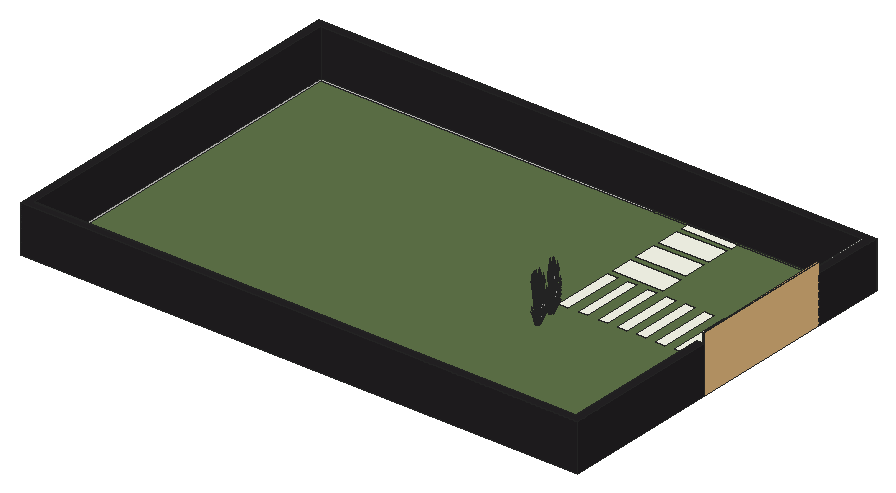
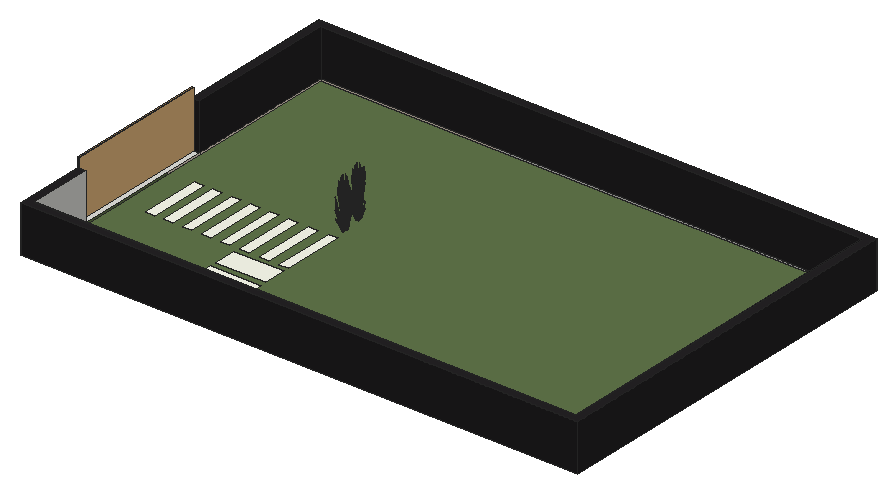
# SketchUp Ruby script. Lengths in inches.
U = 1.inch
M = Sketchup.active_model
def pt(a) = Geom::Point3d.new(a.map { |v| v * U })
def face(e, loops, mat)
  f = e.add_face(loops[0].map { |a| pt(a) })
  loops[1..].each { |l| e.add_face(l.map { |a| pt(a) }).erase! }
  f.material = f.back_material = mat if mat
  f
end
# faces: each face lists its corners as indices into pts; further lists are holes
def faces(e, pts, list, mat = nil) = list.each { |f| face(e, (f[0].is_a?(Array) ? f : [f]).map { |l| l.map { |i| pts[i] } }, mat) }
# xy, xz, yz: faces in a plane at the given z, y or x. An outline is a flat list of corners, or four numbers for a rectangle; further outlines are holes
def ring(l) = l.size == 4 ? [[l[0], l[1]], [l[2], l[1]], [l[2], l[3]], [l[0], l[3]]] : l.each_slice(2).to_a
def flat(e, list, mat, &to3) = list.each { |f| face(e, (f[0].is_a?(Array) ? f : [f]).map { |l| ring(l).map { |u, v| to3.(u, v) } }, mat) }
def xy(e, z, list, mat = nil) = flat(e, list, mat) { |x, y| [x, y, z] }
def xz(e, y, list, mat = nil) = flat(e, list, mat) { |x, z| [x, y, z] }
def yz(e, x, list, mat = nil) = flat(e, list, mat) { |y, z| [x, y, z] }
def lines(e, pts, list) = list.each { |a, b| e.add_line(pt(pts[a]), pt(pts[b])) }
# prism: a flat outline (further loops are holes) pulled along v
def prism(e, loops, v, mat = nil)
  f = face(e, loops, mat); d = Geom::Vector3d.new(v.map { |x| x * U })
  f.pushpull(f.normal.samedirection?(d) ? d.length : -d.length)
end
def box(e, o, s, mat = nil) = prism(e, [[o, [o[0] + s[0], o[1], o[2]], [o[0] + s[0], o[1] + s[1], o[2]], [o[0], o[1] + s[1], o[2]]]], [0, 0, s[2]], mat)
def at(x, y, z, deg = 0) = Geom::Transformation.translation(pt([x, y, z])) * Geom::Transformation.rotation(ORIGIN, Z_AXIS, deg.degrees)
def axes(o, x, y, z) = Geom::Transformation.new([*x, 0, *y, 0, *z, 0, *pt(o).to_a, 1])
def part(name) = M.definitions.add(name)
# library, detail: a bought-in or finely detailed component or shape, given as its bounding box
def library(name, o, s) = part(name).tap { |d| box(d.entities, o, s) }
def detail(e, o, s) = box(e.add_group.entities, o, s)
def put(e, d, t, mat = nil) = e.add_instance(d, t).tap { |i| i.material = mat if mat }
def group(e, t, mat = nil) = e.add_group.tap { |g| g.transformation = t; g.material = mat if mat }.entities
root = M.entities
M.materials.add("Concrete_04_1K").color = [254, 255, 241]
M.materials.add("LightPink_Translucent").color = [144, 107, 117]
M.materials["LightPink_Translucent"].alpha = 0.75
M.materials.add("Marble_07_1K").color = [36, 34, 36]
M.materials.add("Roofing_01_1K1").color = [234, 220, 203]
M.materials.add("Roofing_02_1K").color = [97, 118, 74]
c1 = part("blade")
p = [[2.15,0.21,22],[0,0.17,0],[0.09,0.45,0],[2.18,0.31,22],[2.29,0.31,22],[0.38,0.45,0],
  [2.48,0.24,33],[2.49,0.24,33],[2.48,0.22,33]]
faces(c1.entities,p,[[0,1,2,3],[4,5,2,3],[6,3,4,7],[8,0,3,6]])
c2 = part("seeds")
p = [[0.3,-0.1,1.38],[-0.01,-0.03,1.59],[-0.01,-0.03,0.03],[0.14,-0.07,-0.07],[0.29,-0.03,3],[0.15,0.01,3.11]]
faces(c2.entities,p,[[0,1,2,3],[1,0,4,5]],"LightPink_Translucent")
c3 = part("blade with seeds")
put(c3.entities,c1,at(0,0,0))
put(c3.entities,c2,axes([2.4,0.25,30.99],[1.5799,-0.05474,1.17369],[-0.12525,1.92788,0.29478],[-0.07173,-0.02425,1.56792]))
c4 = library("Modern+Gate+1",[0,0,0],[118.11,1.97,78.74])
xy(root,-4,[[9,9,621,413.18]],"Roofing_02_1K")
xy(root,-2,[[0,0,0,422.18,630,422.18,630,341.02,621,341.02,621,413.18,9,413.18,9,9,621,9,621,179.2,630,179.2,630,0],[621,179.2,630,341.02]])
xy(root,0,[[428.41,225.85,438.8125,295.18],[450.39,225.85,460.8,295.18],[473.09,225.85,483.5,295.18],[494.45,225.85,504.85,295.18],[515.86,225.85,526.26,295.18],
  [537.75,225.85,548.15,295.18],[559.25,225.85,569.66,295.18],[579.86,225.85,590.27,295.18],[428.21,302.1,484.72,327.6],[428.21,335.07,484.72,360.33],
  [428.21,367.55,484.72,392.98],[428.21,399.17,484.72,408.11]],"Concrete_04_1K")
xy(root,51,[[0,0,630,0,630,179.2,621,179.2,621,9,9,9,9,413.18,621,413.18,621,341.02,630,341.02,630,422.18,0,422.18]],"Marble_07_1K")
xz(root,0,[[0,-2,630,51]],"Marble_07_1K")
xz(root,9,[[9,-4,423,-2]])
xz(root,9,[[9,-2,621,51]],"Marble_07_1K")
xz(root,9,[[423,-4,621,-2]],"Roofing_01_1K1")
xz(root,179.2,[[621,-2,630,51]],"Marble_07_1K")
xz(root,341.02,[[621,-2,630,51]],"Marble_07_1K")
xz(root,413.18,[[9,-4,387,-2]])
xz(root,413.18,[[9,-2,621,51]],"Marble_07_1K")
xz(root,413.18,[[387,-4,621,-2]],"Roofing_02_1K")
xz(root,422.18,[[0,-2,630,51]],"Marble_07_1K")
yz(root,0,[[0,-2,422.18,51]],"Marble_07_1K")
yz(root,9,[[9,-4,413.18,-2]])
yz(root,9,[[9,-2,413.18,51]],"Marble_07_1K")
yz(root,621,[[341.02,-2,413.18,51]])
yz(root,621,[[9,-2,179.2,51]],"Marble_07_1K")
yz(root,621,[[9,-4,179.2,-2],[179.2,-4,225.85,-2]],"Roofing_01_1K1")
yz(root,621,[[225.85,-4,294.89,-2],[294.89,-4,341.02,-2],[341.02,-4,413.18,-2]],"Roofing_02_1K")
yz(root,630,[[0,-2,179.2,51],[341.02,-2,422.18,51]],"Marble_07_1K")
put(root,c3,axes([435.76,185.8,0.29],[-0.04385,-0.62963,-0.25022],[0.45669,-0.03807,-0.43002],[0.08042,-0.08387,1.37348]))
put(root,c3,axes([434.63,185.83,-0.26],[0.26266,-0.34428,-0.26641],[0.26266,0.34428,0.26641],[0,-0.11089,1.19518]))
put(root,c3,axes([434.52,184.18,-0.17],[-0.10855,0.45057,-0.03348],[-0.33409,-0.1386,-0.15179],[-0.05073,-0.0737,0.50065]))
put(root,c3,axes([435.55,186.45,0.29],[-0.42377,-0.26329,-0.25022],[0.20405,-0.55571,-0.43002],[-0.01332,-0.13644,1.37348]))
put(root,c3,axes([434.34,186.23,0.04],[-0.47052,0,0],[0,-0.61671,-0.44382],[0,-0.14046,1.40792]))
put(root,c3,axes([435.7,184.4,-0.26],[0.35106,0.13653,-0.26641],[-0.08839,0.48081,0.26641],[0.07077,-0.05545,1.19518]))
put(root,c3,axes([434.71,186.07,0],[-0.35001,0.46392,0.2645],[-0.35022,-0.45904,-0.31383],[-0.01222,-0.13174,1.41801]))
put(root,c3,axes([435.82,186.29,0.09],[0.42398,0.26744,0.20696],[-0.20405,0.55571,0.43002],[0,-0.1281,1.38067]))
put(root,c3,axes([435.66,187.04,0.1],[0.09973,-0.65385,-0.20149],[0.47288,0.11397,0.44093],[-0.08263,-0.0903,1.34539]))
put(root,c3,axes([433.99,185.59,0.38],[0.24023,-0.03948,0.9878],[-0.15239,0.3479,0.72577],[-0.11872,-0.05219,0.21757]))
put(root,c3,axes([435.68,185.92,0.34],[-0.40861,0.03406,0.38476],[-0.03695,-0.56543,-0.18517],[0.07315,-0.05731,1.23533]))
put(root,c3,axes([434.63,186.33,0.13],[0,0.5518,0.427],[-0.42099,0,0],[0,-0.12568,1.35453]))
put(root,c3,axes([437.58,186.45,2.03],[0.10194,-0.50193,-0.43945],[0.34951,0.17204,-0.34039],[0.14072,-0.04602,0.84085]))
put(root,c3,axes([437.03,184.41,0.04],[0.23526,-0.55293,0],[0.3936,0.30836,-0.44382],[0.08964,0.07023,1.40792]))
put(root,c3,axes([435.62,186.77,-0.1],[-0.22605,-0.46315,-0.38476],[0.34239,-0.32614,0.18517],[-0.07315,-0.05731,1.23533]))
put(root,c3,axes([435.67,186.12,0.03],[0.1636,0.61702,0.39349],[-0.46745,0.21456,0.15441],[0.00571,-0.11338,1.36617]))
put(root,c3,axes([437.96,186.59,-0.3],[-0.24235,0.06622,1.21762],[-0.03858,-0.5271,0.0697],[0.16974,-0.07978,0.69287]))
put(root,c3,axes([438.4,186.125,-0.06],[-0.23329,-0.35284,-0.05579],[0.2555,-0.3233,-0.25298],[0.0724,-0.02276,0.83441]))
put(root,c3,axes([435.59,186.61,0.34],[-0.18257,0.49721,0.38476],[-0.37935,-0.23929,-0.18517],[0,-0.11462,1.23533]))
put(root,c3,axes([436.26,186.17,-0.1],[0,-0.63847,0],[0.47052,0,0],[0,0,1.54332]))
put(root,c3,axes([436.83,184.7,0.13],[-0.35217,-0.2759,0.427],[0.2105,-0.49473,0],[0.08021,0.06284,1.35453]))
put(root,c3,axes([437.52,186.63,2.28],[0.33065,-0.2437,-0.61099],[0.18427,0.50165,0.07373],[0.15976,-0.05699,0.8643]))
put(root,c3,axes([435.42,186.95,-0.23],[-0.39143,-0.09047,-0.53624],[0.0826,-0.55804,-0.14074],[-0.11681,-0.06762,1.18365]))
put(root,c3,axes([436.04,185.77,0.03],[-0.312,0.50076,0.39349],[-0.37066,-0.44204,0.15441],[0.07522,-0.04998,1.36617]))
put(root,c3,axes([436.375,186.67,-0.02],[-0.35001,-0.47494,-0.05273],[0.35022,-0.47523,0],[-0.01222,-0.01659,1.50991]))
put(root,c3,axes([435.49,184.95,0.13],[-0.1087,0.54839,0.15172],[-0.39778,-0.15519,0.30174],[0.06871,-0.00267,1.3795]))
put(root,c3,axes([435.33,185.39,-0.63],[-0.37038,0.22092,1.10879],[-0.11789,-0.63387,0.43083],[0.22743,0.01055,1.26112]))
put(root,c3,axes([436.32,185.55,0.25],[0.07259,-0.49245,0.12452],[0.35466,0.08548,-0.35559],[0.06454,0.05057,1.09]))
put(root,c3,axes([435.71,186.72,0.03],[0.4756,0.11626,0.39349],[-0.09679,0.6566,0.15441],[-0.0695,-0.0634,1.36617]))
put(root,c3,axes([438.22,186.25,-0.72],[-0.01967,-0.08377,1.51654],[0.1364,-0.49004,-0.23168],[0.13759,-0.00705,0.25832]))
put(root,c3,axes([436.17,185.68,0.34],[-0.22605,-0.46315,0.38476],[0.34239,-0.32614,-0.18517],[0.07315,0.05731,1.23533]))
put(root,c3,axes([435,187.8,-0.26],[-0.08839,-0.48081,-0.26641],[0.35106,-0.13653,0.26641],[-0.07077,-0.05545,1.19518]))
put(root,c3,axes([435.46,187.77,0.13],[0.40434,-0.14646,0.15172],[0.09984,0.54504,0.30174],[-0.03606,-0.07941,1.3795]))
put(root,c3,axes([436.29,185.71,0.29],[0.37992,-0.36634,-0.25022],[0.25264,0.51764,-0.43002],[0.09374,0.05257,1.37348]))
put(root,c3,axes([437.8,186.68,1.89],[0.31272,0.15393,-0.30456],[-0.09121,0.44909,0.39319],[0.1259,-0.04118,0.75234]))
put(root,c3,axes([434.91,188.01,-0.26],[-0.35217,-0.2759,-0.427],[0.2105,-0.49473,0],[-0.08021,-0.06284,1.35453]))
put(root,c3,axes([437.25,184.74,-0.26],[0.35217,0.2759,-0.427],[-0.2105,0.49473,0],[0.08021,0.06284,1.35453]))
put(root,c3,axes([436.58,186.31,-0.1],[0.42099,0,0],[0,0.57126,0],[0,0,1.5343]))
put(root,c3,axes([435.86,187.03,0.29],[-0.37992,0.36634,-0.25022],[-0.25264,-0.51764,-0.43002],[-0.09374,-0.05257,1.37348]))
put(root,c3,axes([436.7,184.98,0.13],[-0.40434,0.14646,0.15172],[-0.09984,-0.54504,0.30174],[0.03606,0.07941,1.3795]))
put(root,c3,axes([437.15,184.95,-0.26],[0.08839,0.48081,-0.26641],[-0.35106,0.13653,0.26641],[0.07077,0.05545,1.19518]))
put(root,c3,axes([436.44,186.02,0.05],[-0.4756,-0.11626,0.42311],[0.09679,-0.6566,0.16603],[0.0695,0.0634,1.46899]))
put(root,c3,axes([436.0625,187.64,-0.1],[-0.12277,-0.47573,0],[0.35059,-0.1666,0],[0,0,1.32759]))
put(root,c3,axes([435.83,187.19,0.25],[-0.07259,0.49245,0.12452],[-0.35466,-0.08548,-0.35559],[-0.06454,-0.05057,1.09]))
put(root,c3,axes([436.52,187.58,-0.12],[0.39505,-0.18722,-0.1651],[0.13882,0.53931,0.00007],[0.04361,-0.02069,1.49552]))
put(root,c3,axes([436.66,187.8,0.13],[0.1087,-0.54839,0.15172],[0.39778,0.15519,0.30174],[-0.06871,0.00267,1.3795]))
put(root,c3,axes([436.57,186.56,-0.1],[0.26266,0.35642,0],[-0.26266,0.35642,0],[0,0,1.45569]))
put(root,c3,axes([437.28,186.4,0.13],[-0.29564,-0.40194,0.15172],[0.29793,-0.38985,0.30174],[-0.03265,0.08208,1.3795]))
put(root,c3,axes([436.73,185.8,-0.23],[0.39143,0.09047,-0.53624],[-0.0826,0.55804,-0.14074],[0.11681,0.06762,1.18365]))
put(root,c3,axes([438.46,186.77,0.38],[-0.23249,0.0911,0.9878],[0.10944,-0.37648,0.72577],[0.12334,0.02576,0.21757]))
put(root,c3,axes([435.98,187.86,-0.11],[-0.37935,-0.24773,0],[0.18257,-0.51475,0],[0,0,1.39928]))
put(root,c3,axes([436.29,187.2,0.12],[-0.36743,-0.44413,-0.21665],[0.30918,-0.49872,0.47412],[-0.09894,0.05195,1.44665]))
put(root,c3,axes([435.32,188.05,0.13],[0.35217,0.2759,0.427],[-0.2105,0.49473,0],[-0.08021,-0.06284,1.35453]))
put(root,c3,axes([436.5625,186.14,0.34],[0.18257,-0.49721,0.38476],[0.37935,0.23929,-0.18517],[0,0.11462,1.23533]))
put(root,c3,axes([436.49,186.43,-0.03],[0,0.63816,-0.04848],[-0.47052,0,0],[0,0.02005,1.54256]))
put(root,c3,axes([436.53,185.97,-0.1],[0.22605,0.46315,-0.38476],[-0.34239,0.32614,0.18517],[0.07315,0.05731,1.23533]))
put(root,c3,axes([435.12,188.34,0.04],[-0.23526,0.55293,0],[-0.3936,-0.30836,-0.44382],[-0.08964,-0.07023,1.40792]))
put(root,c3,axes([437.52,186.42,0.13],[0,-0.5518,0.427],[0.42099,0,0],[0,0.12568,1.35453]))
put(root,c3,axes([436.47,186.83,0.34],[0.40861,-0.03406,0.38476],[0.03695,0.56543,-0.18517],[-0.07315,0.05731,1.23533]))
put(root,c3,axes([436.72,186.26,0.25],[0.35059,-0.16092,0.12452],[0.12277,0.45952,-0.35559],[0,0.10113,1.09]))
put(root,c3,axes([436.1,187.11,-0.1],[-0.40861,0.03406,-0.38476],[-0.03695,-0.56543,0.18517],[-0.07315,0.05731,1.23533]))
put(root,c3,axes([438.03,187.375,0.23],[-0.09062,-0.13571,1.22981],[0.11791,-0.44895,-0.26449],[0.18335,0.06082,0.52581]))
put(root,c3,axes([436.41,187.87,-0.1],[0.37935,0.24773,0],[-0.18257,0.51475,0],[0,0,1.5046]))
put(root,c3,axes([436.56,188.42,-0.11],[-0.23233,-0.55486,-0.04422],[0.3936,-0.30836,0.44382],[-0.09699,0.05283,1.40722]))
put(root,c3,axes([436.47,187.08,0.25],[0.278,0.33153,0.12452],[-0.23189,0.37404,-0.35559],[-0.06454,0.05057,1.09]))
put(root,c3,axes([437.19,187.65,2.28],[0.37615,0.01329,-0.61099],[-0.02526,0.55946,0.07373],[0.15935,0.05904,0.8643]))
put(root,c3,axes([436.77,188.1,0.13],[0.35217,-0.2759,0.427],[0.2105,0.49473,0],[-0.08021,0.06284,1.35453]))
put(root,c3,axes([436.27,187.66,-0.03],[0.1636,0.63392,-0.05171],[-0.46745,0.22213,0],[0.00571,0.02214,1.48069]))
put(root,c3,axes([436.45,188.35,-0.26],[-0.35106,-0.13653,-0.26641],[0.08839,-0.48081,0.26641],[-0.07077,0.05545,1.19518]))
put(root,c3,axes([437.81,186.51,0.04],[0.47052,0,0],[0,0.61671,-0.44382],[0,0.14046,1.40792]))
put(root,c3,axes([437.62,186.83,-0.11],[-0.47029,-0.00441,-0.0428],[0,-0.61671,0.42951],[-0.01478,0.14039,1.36183]))
put(root,c3,axes([436.6,186.29,0.29],[0.42377,0.26329,-0.25022],[-0.20405,0.55571,-0.43002],[0.01332,0.13644,1.37348]))
put(root,c3,axes([433.65,188.34,0.38],[0.15682,-0.25009,0.9878],[0.06188,0.39591,0.72577],[-0.11333,0.07089,0.21757]))
put(root,c3,axes([437.42,187.88,1.89],[0.2141,0.34548,-0.30456],[-0.24447,0.32704,0.39319],[0.12421,0.04976,0.75234]))
put(root,c3,axes([437.52,186.92,-0.26],[-0.26266,0.34428,-0.26641],[-0.26266,-0.34428,0.26641],[0,0.11089,1.19518]))
put(root,c3,axes([436.39,186.95,0.29],[0.04385,0.62963,-0.25022],[-0.45669,0.03807,-0.43002],[-0.08042,0.08387,1.37348]))
put(root,c3,axes([436.56,186.71,-0.1],[-0.18257,0.49721,-0.38476],[-0.37935,-0.23929,0.18517],[0,0.11462,1.23533]))
put(root,c3,axes([434.24,187.26,1.89],[-0.32754,0.07886,-0.30456],[-0.08649,-0.45081,0.39319],[-0.09386,0.12109,0.75234]))
put(root,c3,axes([436.12,187.43,-0.23],[-0.25345,0.41475,-0.53624],[-0.31485,-0.37608,-0.14074],[-0.10156,0.10346,1.18365]))
put(root,c3,axes([436.57,188.13,0],[0.47108,0.17935,0.2645],[-0.11785,0.64108,-0.31383],[-0.07797,0.08023,1.41801]))
put(root,c3,axes([436.53,188.57,-0.26],[-0.35217,0.2759,-0.427],[-0.2105,-0.49473,0],[-0.08021,0.06284,1.35453]))
put(root,c3,axes([437.7,186.93,-0.26],[0,0.5518,-0.427],[-0.42099,0,0],[0,0.12568,1.35453]))
put(root,c3,axes([437.17,188.08,0.38],[-0.21187,-0.15866,0.9878],[0.27357,-0.16121,0.72577],[0.07379,0.13656,0.21757]))
put(root,c3,axes([434.51,187.3125,2.03],[0.09666,0.50384,-0.43945],[-0.36608,0.08814,-0.34039],[-0.10491,0.13533,0.84085]))
put(root,c3,axes([436.85,188.48,0.04],[0.23526,0.55293,0],[-0.3936,0.30836,-0.44382],[-0.08964,0.07023,1.40792]))
put(root,c3,axes([437.23,188.67,-0.72],[0.02741,-0.07966,1.51654],[0.34514,-0.23462,-0.23168],[0.10464,0.12143,0.25832]))
put(root,c3,axes([436.65,186.29,0.44],[-0.01028,-0.51954,1.21494],[0.46521,0.13467,0.51441],[-0.11003,0.28429,1.14681]))
put(root,c3,axes([436.77,186.86,-0.2],[0.13798,0.50522,-0.59522],[-0.39745,0.18195,-0.15622],[0.01525,0.17108,1.31385]))
put(root,c3,axes([434.06,188.6,-0.72],[0.05047,0.05513,1.51654],[0.08558,0.51079,-0.23168],[-0.11187,0.10892,0.25832]))
put(root,c3,axes([436.69,188.3,2.03],[0.37131,-0.13117,-0.43945],[0.06495,0.49674,-0.34039],[0.09973,0.14235,0.84085]))
put(root,c3,axes([437.2,188.8,0.29],[-0.2413,-0.01731,0.90352],[0.15935,-0.36755,0.49885],[0.09532,0.13058,0.70873]))
put(root,c3,axes([436.41,187.91,0.23],[0.00664,-0.18292,1.22981],[0.31732,-0.20432,-0.26449],[0.09796,0.21893,0.52581]))
put(root,c3,axes([434.8125,188.3,1.89],[-0.2546,0.29052,-0.30456],[-0.24101,-0.33173,0.39319],[-0.03667,0.16855,0.75234]))
put(root,c3,axes([434.98,189.43,0.38],[-0.00974,-0.3281,0.9878],[0.24334,0.23402,0.72577],[-0.04786,0.15639,0.21757]))
put(root,c3,axes([435.62,188.65,-0.72],[0.0609,-0.03003,1.51654],[0.36632,0.16527,-0.23168],[0.01071,0.18627,0.25832]))
put(root,c3,axes([435.07,188.17,2.3],[0.26937,0.37076,-0.48779],[-0.28456,0.3247,-0.37783],[-0.04099,0.18838,0.93334]))
put(root,c3,axes([434.77,188.72,0.43],[0.34184,-0.09771,0.05596],[0.07859,0.39367,-0.74222],[-0.02167,0.19928,0.6653]))
put(root,c3,axes([435.87,188.53,2.03],[0.3699,0.13833,-0.43945],[-0.12679,0.47426,-0.34039],[0.03392,0.19095,0.84085]))
put(root,c3,axes([435.7,188.82,1.89],[-0.11344,0.42434,-0.30456],[-0.33096,-0.12377,0.39319],[0.03035,0.17085,0.75234]))
put(root,c3,axes([434.98,188,2.59],[-0.00979,0.51041,-0.6782],[-0.4123,-0.03428,0.08184],[-0.04351,0.21623,0.95938]))
put(root,c3,axes([435.73,188.4375,2.28],[0.17959,0.44867,-0.61099],[-0.36969,0.25004,0.07373],[0.042,0.21679,0.8643]))
put(root,c3,axes([434.69,189.14,0.23],[0.11874,-0.08705,1.22981],[0.29317,0.26247,-0.26449],[-0.08726,0.22711,0.52581]))
put(root,c3,axes([434.84,188.72,0.89],[0.00827,-0.28486,1.32737],[0.37184,0.15046,0.18343],[-0.03222,0.30359,0.62678]))
put(root,c3,axes([433.22,207.92,0.23],[-0.10696,0.11169,1.22981],[-0.32033,-0.19549,-0.26449],[0.05938,-0.24312,0.52581]))
put(root,c3,axes([432.74,208.31,2.28],[-0.17959,-0.44867,-0.61099],[0.36969,-0.25004,0.07373],[-0.042,-0.21679,0.8643]))
put(root,c3,axes([432.43,207.3125,-0.72],[-0.06312,0.01988,1.51654],[-0.34903,-0.22379,-0.23168],[0.00586,-0.18666,0.25832]))
put(root,c3,axes([433.48,208.75,2.28],[0.00979,-0.51041,-0.61099],[0.4123,0.03428,0.07373],[0.04351,-0.21623,0.8643]))
put(root,c3,axes([432.83,207.03,0.38],[0.04827,0.32177,0.9878],[-0.26778,-0.17821,0.72577],[0.02882,-0.16476,0.21757]))
put(root,c3,axes([433.4,208.58,2.03],[-0.26937,-0.37076,-0.43945],[0.28456,-0.3247,-0.34039],[0.04099,-0.18838,0.84085]))
put(root,c3,axes([433.97,208.26,-0.72],[-0.05632,-0.04347,1.51654],[-0.14467,-0.48565,-0.23168],[0.09759,-0.13179,0.25832]))
put(root,c3,axes([433.97,209.63,2.28],[0.19655,-0.43539,-0.61099],[0.34443,0.30942,0.07373],[0.11736,-0.15774,0.8643]))
put(root,c3,axes([431.84,208.37,0.04],[-0.23526,-0.55293,0],[0.3936,-0.30836,-0.44382],[0.08964,-0.07023,1.40792]))
put(root,c3,axes([433.96,209.43,2.03],[-0.09666,-0.50384,-0.43945],[0.36608,-0.08814,-0.34039],[0.10491,-0.13533,0.84085]))
put(root,c3,axes([432.16,208.28,-0.26],[0.35217,-0.2759,-0.427],[0.2105,0.49473,0],[0.08021,-0.06284,1.35453]))
put(root,c3,axes([434.25,209.23,0.23],[-0.13443,-0.01634,1.22981],[-0.13772,-0.43844,-0.26449],[0.16514,-0.12403,0.52581]))
put(root,c3,axes([432.58,209.41,-0.23],[0.25345,-0.41475,-0.53624],[0.31485,0.37608,-0.14074],[0.10156,-0.10346,1.18365]))
put(root,c3,axes([434.41,208.43,0.38],[-0.12533,0.28089,0.9878],[-0.10773,-0.37739,0.72577],[0.10352,-0.09457,0.21757]))
put(root,c3,axes([432.14,210.14,-0.1],[0.18257,-0.49721,-0.38476],[0.37935,0.23929,0.18517],[0,-0.11462,1.23533]))
put(root,c3,axes([432.31,209.89,0.29],[-0.04385,-0.62963,-0.25022],[0.45669,-0.03807,-0.43002],[0.08042,-0.08387,1.37348]))
put(root,c3,axes([432.25,208.5,-0.26],[0.35106,0.13653,-0.26641],[-0.08839,0.48081,0.26641],[0.07077,-0.05545,1.19518]))
put(root,c3,axes([432.37,210.39,0.09],[0.42398,0.26744,0.20696],[-0.20405,0.55571,0.43002],[0,-0.1281,1.38067]))
put(root,c3,axes([432.23,210.01,0.34],[-0.40861,0.03406,0.38476],[-0.03695,-0.56543,-0.18517],[0.07315,-0.05731,1.23533]))
put(root,c3,axes([434.13,210.55,2.03],[0.10194,-0.50193,-0.43945],[0.34951,0.17204,-0.34039],[0.14072,-0.04602,0.84085]))
put(root,c3,axes([433.58,208.51,0.04],[0.23526,-0.55293,0],[0.3936,0.30836,-0.44382],[0.08964,0.07023,1.40792]))
put(root,c3,axes([432.22,210.22,0.03],[0.1636,0.61702,0.39349],[-0.46745,0.21456,0.15441],[0.00571,-0.11338,1.36617]))
put(root,c3,axes([434.5,210.69,-0.3],[-0.24235,0.06622,1.21762],[-0.03858,-0.5271,0.0697],[0.16974,-0.07978,0.69287]))
put(root,c3,axes([434.94,210.22,-0.06],[-0.23329,-0.35284,-0.05579],[0.2555,-0.3233,-0.25298],[0.0724,-0.02276,0.83441]))
put(root,c3,axes([432.8,210.27,-0.1],[0,-0.63847,0],[0.47052,0,0],[0,0,1.54332]))
put(root,c3,axes([433.375,208.79,0.13],[-0.35217,-0.2759,0.427],[0.2105,-0.49473,0],[0.08021,0.06284,1.35453]))
put(root,c3,axes([434.0625,210.73,2.28],[0.33065,-0.2437,-0.61099],[0.18427,0.50165,0.07373],[0.15976,-0.05699,0.8643]))
put(root,c3,axes([432.58,209.87,0.03],[-0.312,0.50076,0.39349],[-0.37066,-0.44204,0.15441],[0.07522,-0.04998,1.36617]))
put(root,c3,axes([432.92,210.76,-0.02],[-0.35001,-0.47494,-0.05273],[0.35022,-0.47523,0],[-0.01222,-0.01659,1.50991]))
put(root,c3,axes([432.04,209.04,0.13],[-0.1087,0.54839,0.15172],[-0.39778,-0.15519,0.30174],[0.06871,-0.00267,1.3795]))
put(root,c3,axes([431.875,209.49,-0.63],[-0.37038,0.22092,1.10879],[-0.11789,-0.63387,0.43083],[0.22743,0.01055,1.26112]))
put(root,c3,axes([432.87,209.65,0.25],[0.07259,-0.49245,0.12452],[0.35466,0.08548,-0.35559],[0.06454,0.05057,1.09]))
put(root,c3,axes([434.77,210.35,-0.72],[-0.01967,-0.08377,1.51654],[0.1364,-0.49004,-0.23168],[0.13759,-0.00705,0.25832]))
put(root,c3,axes([432.72,209.78,0.34],[-0.22605,-0.46315,0.38476],[0.34239,-0.32614,-0.18517],[0.07315,0.05731,1.23533]))
put(root,c3,axes([432,211.87,0.13],[0.40434,-0.14646,0.15172],[0.09984,0.54504,0.30174],[-0.03606,-0.07941,1.3795]))
put(root,c3,axes([432.83,209.8125,0.29],[0.37992,-0.36634,-0.25022],[0.25264,0.51764,-0.43002],[0.09374,0.05257,1.37348]))
put(root,c3,axes([433.79,208.84,-0.26],[0.35217,0.2759,-0.427],[-0.2105,0.49473,0],[0.08021,0.06284,1.35453]))
put(root,c3,axes([433.12,210.41,-0.1],[0.42099,0,0],[0,0.57126,0],[0,0,1.5343]))
put(root,c3,axes([433.24,209.07,0.13],[-0.40434,0.14646,0.15172],[-0.09984,-0.54504,0.30174],[0.03606,0.07941,1.3795]))
put(root,c3,axes([433.69,209.04,-0.26],[0.08839,0.48081,-0.26641],[-0.35106,0.13653,0.26641],[0.07077,0.05545,1.19518]))
put(root,c3,axes([432.99,210.12,0.05],[-0.4756,-0.11626,0.42311],[0.09679,-0.6566,0.16603],[0.0695,0.0634,1.46899]))
put(root,c3,axes([432.61,211.74,-0.1],[-0.12277,-0.47573,0],[0.35059,-0.1666,0],[0,0,1.32759]))
put(root,c3,axes([433.07,211.68,-0.12],[0.39505,-0.18722,-0.1651],[0.13882,0.53931,0.00007],[0.04361,-0.02069,1.49552]))
put(root,c3,axes([433.2,211.9,0.13],[0.1087,-0.54839,0.15172],[0.39778,0.15519,0.30174],[-0.06871,0.00267,1.3795]))
put(root,c3,axes([433.11,210.66,-0.1],[0.26266,0.35642,0],[-0.26266,0.35642,0],[0,0,1.45569]))
put(root,c3,axes([433.82,210.5,0.13],[-0.29564,-0.40194,0.15172],[0.29793,-0.38985,0.30174],[-0.03265,0.08208,1.3795]))
put(root,c3,axes([433.28,209.89,-0.23],[0.39143,0.09047,-0.53624],[-0.0826,0.55804,-0.14074],[0.11681,0.06762,1.18365]))
put(root,c3,axes([435.01,210.87,0.38],[-0.23249,0.0911,0.9878],[0.10944,-0.37648,0.72577],[0.12334,0.02576,0.21757]))
put(root,c3,axes([432.52,211.96,-0.11],[-0.37935,-0.24773,0],[0.18257,-0.51475,0],[0,0,1.39928]))
put(root,c3,axes([433.11,210.24,0.34],[0.18257,-0.49721,0.38476],[0.37935,0.23929,-0.18517],[0,0.11462,1.23533]))
put(root,c3,axes([433.04,210.52,-0.03],[0,0.63816,-0.04848],[-0.47052,0,0],[0,0.02005,1.54256]))
put(root,c3,axes([433.07,210.07,-0.1],[0.22605,0.46315,-0.38476],[-0.34239,0.32614,0.18517],[0.07315,0.05731,1.23533]))
put(root,c3,axes([434.07,210.52,0.13],[0,-0.5518,0.427],[0.42099,0,0],[0,0.12568,1.35453]))
put(root,c3,axes([433.01,210.93,0.34],[0.40861,-0.03406,0.38476],[0.03695,0.56543,-0.18517],[-0.07315,0.05731,1.23533]))
put(root,c3,axes([433.27,210.35,0.25],[0.35059,-0.16092,0.12452],[0.12277,0.45952,-0.35559],[0,0.10113,1.09]))
put(root,c3,axes([434.57,211.47,0.23],[-0.09062,-0.13571,1.22981],[0.11791,-0.44895,-0.26449],[0.18335,0.06082,0.52581]))
put(root,c3,axes([432.95,211.97,-0.1],[0.37935,0.24773,0],[-0.18257,0.51475,0],[0,0,1.5046]))
put(root,c3,axes([433.02,211.17,0.25],[0.278,0.33153,0.12452],[-0.23189,0.37404,-0.35559],[-0.06454,0.05057,1.09]))
put(root,c3,axes([433.74,211.75,2.28],[0.37615,0.01329,-0.61099],[-0.02526,0.55946,0.07373],[0.15935,0.05904,0.8643]))
put(root,c3,axes([433.32,212.19,0.13],[0.35217,-0.2759,0.427],[0.2105,0.49473,0],[-0.08021,0.06284,1.35453]))
put(root,c3,axes([432.81,211.76,-0.03],[0.1636,0.63392,-0.05171],[-0.46745,0.22213,0],[0.00571,0.02214,1.48069]))
put(root,c3,axes([434.35,210.61,0.04],[0.47052,0,0],[0,0.61671,-0.44382],[0,0.14046,1.40792]))
put(root,c3,axes([434.17,210.93,-0.11],[-0.47029,-0.00441,-0.0428],[0,-0.61671,0.42951],[-0.01478,0.14039,1.36183]))
put(root,c3,axes([433.15,210.39,0.29],[0.42377,0.26329,-0.25022],[-0.20405,0.55571,-0.43002],[0.01332,0.13644,1.37348]))
put(root,c3,axes([434.07,211.02,-0.26],[-0.26266,0.34428,-0.26641],[-0.26266,-0.34428,0.26641],[0,0.11089,1.19518]))
put(root,c3,axes([433.1,210.8,-0.1],[-0.18257,0.49721,-0.38476],[-0.37935,-0.23929,0.18517],[0,0.11462,1.23533]))
put(root,c3,axes([433.11,212.23,0],[0.47108,0.17935,0.2645],[-0.11785,0.64108,-0.31383],[-0.07797,0.08023,1.41801]))
put(root,c3,axes([434.25,211.03,-0.26],[0,0.5518,-0.427],[-0.42099,0,0],[0,0.12568,1.35453]))
put(root,c3,axes([433.71,212.17,0.38],[-0.21187,-0.15866,0.9878],[0.27357,-0.16121,0.72577],[0.07379,0.13656,0.21757]))
put(root,c3,axes([433.4,212.58,0.04],[0.23526,0.55293,0],[-0.3936,0.30836,-0.44382],[-0.08964,0.07023,1.40792]))
put(root,c3,axes([433.77,212.76,-0.72],[0.02741,-0.07966,1.51654],[0.34514,-0.23462,-0.23168],[0.10464,0.12143,0.25832]))
put(root,c3,axes([433.32,210.95,-0.2],[0.13798,0.50522,-0.59522],[-0.39745,0.18195,-0.15622],[0.01525,0.17108,1.31385]))
put(root,c3,axes([433.24,212.39,2.03],[0.37131,-0.13117,-0.43945],[0.06495,0.49674,-0.34039],[0.09973,0.14235,0.84085]))
put(root,c3,axes([433.75,212.9,0.29],[-0.2413,-0.01731,0.90352],[0.15935,-0.36755,0.49885],[0.09532,0.13058,0.70873]))
put(root,c3,axes([432.96,212,0.23],[0.00664,-0.18292,1.22981],[0.31732,-0.20432,-0.26449],[0.09796,0.21893,0.52581]))
put(root,c3,axes([432.16,212.75,-0.72],[0.0609,-0.03003,1.51654],[0.36632,0.16527,-0.23168],[0.01071,0.18627,0.25832]))
put(root,c3,axes([432.41,212.625,2.03],[0.3699,0.13833,-0.43945],[-0.12679,0.47426,-0.34039],[0.03392,0.19095,0.84085]))
put(root,c3,axes([432.28,212.53,2.28],[0.17959,0.44867,-0.61099],[-0.36969,0.25004,0.07373],[0.042,0.21679,0.8643]))
put(root,c4,axes([630,179.2,-2],[0,1.37007,0],[-1,0,0],[0,0,0.81]))
